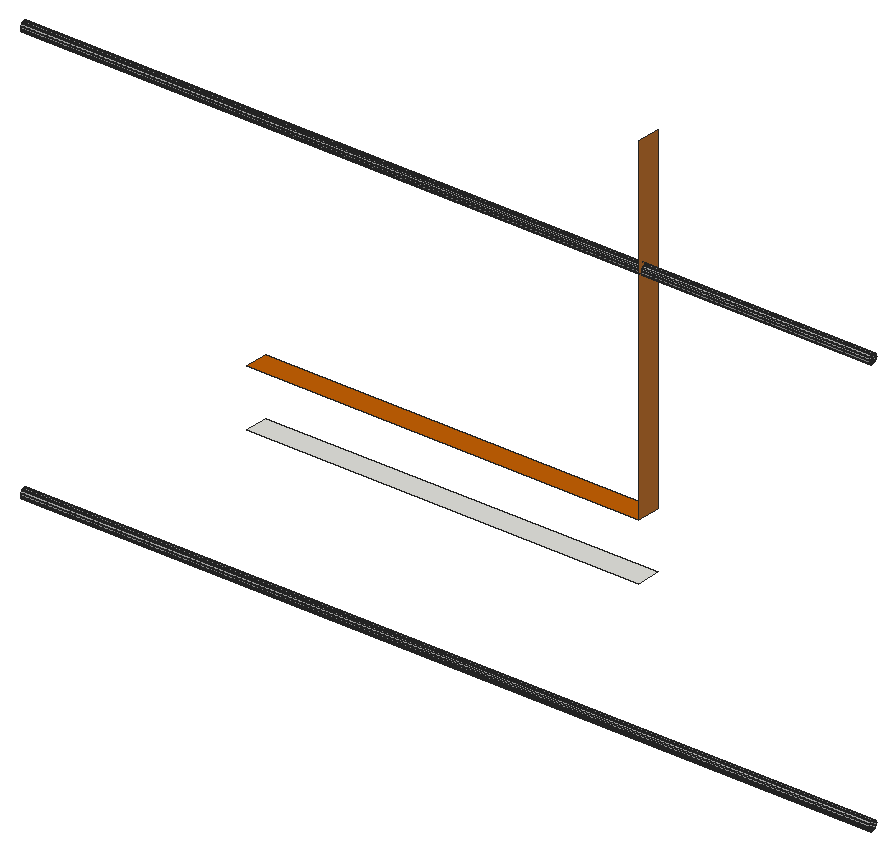
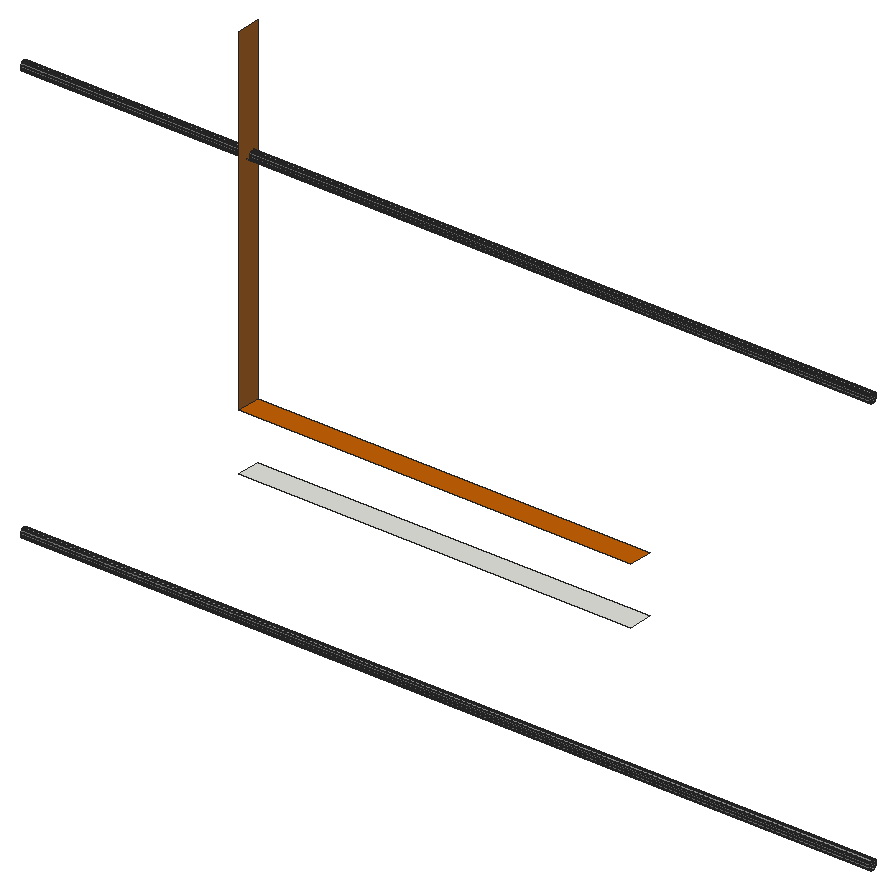
# SketchUp Ruby script. Lengths in inches.
U = 1.inch
M = Sketchup.active_model
def pt(a) = Geom::Point3d.new(a.map { |v| v * U })
def face(e, loops, mat)
  f = e.add_face(loops[0].map { |a| pt(a) })
  loops[1..].each { |l| e.add_face(l.map { |a| pt(a) }).erase! }
  f.material = f.back_material = mat if mat
  f
end
# faces: each face lists its corners as indices into pts; further lists are holes
def faces(e, pts, list, mat = nil) = list.each { |f| face(e, (f[0].is_a?(Array) ? f : [f]).map { |l| l.map { |i| pts[i] } }, mat) }
# xy, xz, yz: faces in a plane at the given z, y or x. An outline is a flat list of corners, or four numbers for a rectangle; further outlines are holes
def ring(l) = l.size == 4 ? [[l[0], l[1]], [l[2], l[1]], [l[2], l[3]], [l[0], l[3]]] : l.each_slice(2).to_a
def flat(e, list, mat, &to3) = list.each { |f| face(e, (f[0].is_a?(Array) ? f : [f]).map { |l| ring(l).map { |u, v| to3.(u, v) } }, mat) }
def xy(e, z, list, mat = nil) = flat(e, list, mat) { |x, y| [x, y, z] }
def xz(e, y, list, mat = nil) = flat(e, list, mat) { |x, z| [x, y, z] }
def yz(e, x, list, mat = nil) = flat(e, list, mat) { |y, z| [x, y, z] }
def lines(e, pts, list) = list.each { |a, b| e.add_line(pt(pts[a]), pt(pts[b])) }
# prism: a flat outline (further loops are holes) pulled along v
def prism(e, loops, v, mat = nil)
  f = face(e, loops, mat); d = Geom::Vector3d.new(v.map { |x| x * U })
  f.pushpull(f.normal.samedirection?(d) ? d.length : -d.length)
end
def box(e, o, s, mat = nil) = prism(e, [[o, [o[0] + s[0], o[1], o[2]], [o[0] + s[0], o[1] + s[1], o[2]], [o[0], o[1] + s[1], o[2]]]], [0, 0, s[2]], mat)
def at(x, y, z, deg = 0) = Geom::Transformation.translation(pt([x, y, z])) * Geom::Transformation.rotation(ORIGIN, Z_AXIS, deg.degrees)
def axes(o, x, y, z) = Geom::Transformation.new([*x, 0, *y, 0, *z, 0, *pt(o).to_a, 1])
def part(name) = M.definitions.add(name)
# library, detail: a bought-in or finely detailed component or shape, given as its bounding box
def library(name, o, s) = part(name).tap { |d| box(d.entities, o, s) }
def detail(e, o, s) = box(e.add_group.entities, o, s)
def put(e, d, t, mat = nil) = e.add_instance(d, t).tap { |i| i.material = mat if mat }
def group(e, t, mat = nil) = e.add_group.tap { |g| g.transformation = t; g.material = mat if mat }.entities
root = M.entities
M.materials.add("[0132_LightGray]").color = [169, 169, 169]
M.materials.add("[Wood Bamboo]").color = [195, 96, 5]
M.materials.add("[Wood Bamboo]1").color = [177, 105, 43]
xy(root,94.9,[[340.01,40.5625,381.26,43]])
xy(root,100.9,[[340.01,40.5625,381.26,43]],"[Wood Bamboo]")
yz(root,381.26,[[40.5625,100.9,43,136.59]],"[Wood Bamboo]1")
p = [[316.01,41.03,79.78],[316.01,41.15,79.73],[405.26,41.15,79.73],[405.26,41.03,79.78],[316.01,41.28,79.71],[405.26,41.28,79.71],
  [316.01,41.41,79.73],[405.26,41.41,79.73],[316.01,41.53,79.78],[405.26,41.53,79.78],[316.01,40.93,79.86],[405.26,40.93,79.86],
  [316.01,41.63,79.86],[405.26,41.63,79.86],[316.01,40.85,79.96],[405.26,40.85,79.96],[316.01,41.71,79.96],[405.26,41.71,79.96],
  [316.01,40.8,80.08],[405.26,40.8,80.08],[316.01,41.76,80.08],[405.26,41.76,80.08],[316.01,40.78,80.21],[405.26,40.78,80.21],
  [316.01,41.78,80.21],[405.26,41.78,80.21],[316.01,40.8,80.34],[405.26,40.8,80.34],[316.01,41.76,80.34],[405.26,41.76,80.34],
  [316.01,40.85,80.46],[405.26,40.85,80.46],[316.01,41.71,80.46],[405.26,41.71,80.46],[316.01,40.93,80.57],[405.26,40.93,80.57],
  [316.01,41.63,80.57],[405.26,41.63,80.57],[316.01,41.03,80.65],[405.26,41.03,80.65],[316.01,41.15,80.7],[405.26,41.15,80.7],
  [316.01,41.53,80.65],[316.01,41.41,80.7],[405.26,41.41,80.7],[405.26,41.53,80.65],[316.01,41.28,80.71],[405.26,41.28,80.71],
  [316.01,41.03,123.78],[316.01,41.15,123.73],[405.26,41.15,123.73],[405.26,41.03,123.78],[316.01,41.28,123.71],[405.26,41.28,123.71],
  [316.01,41.41,123.73],[405.26,41.41,123.73],[316.01,41.53,123.78],[405.26,41.53,123.78],[316.01,40.93,123.86],[405.26,40.93,123.86],
  [316.01,41.63,123.86],[405.26,41.63,123.86],[316.01,40.85,123.96],[405.26,40.85,123.96],[316.01,41.71,123.96],[405.26,41.71,123.96],
  [316.01,40.8,124.08],[405.26,40.8,124.08],[316.01,41.76,124.08],[405.26,41.76,124.08],[316.01,40.78,124.21],[405.26,40.78,124.21],
  [316.01,41.78,124.21],[405.26,41.78,124.21],[316.01,40.8,124.34],[405.26,40.8,124.34],[316.01,41.76,124.34],[405.26,41.76,124.34],
  [316.01,40.85,124.46],[405.26,40.85,124.46],[316.01,41.71,124.46],[405.26,41.71,124.46],[316.01,40.93,124.57],[405.26,40.93,124.57],
  [316.01,41.63,124.57],[405.26,41.63,124.57],[316.01,41.03,124.65],[405.26,41.03,124.65],[316.01,41.15,124.7],[405.26,41.15,124.7],
  [316.01,41.53,124.65],[316.01,41.41,124.7],[405.26,41.41,124.7],[405.26,41.53,124.65],[316.01,41.28,124.71],[405.26,41.28,124.71]]
faces(root,p,[[0,1,2,3],[1,4,5,2],[4,6,7,5],[6,8,9,7],[10,0,3,11],[8,12,13,9],[14,10,11,15],[12,16,17,13],
  [18,14,15,19],[16,20,21,17],[22,18,19,23],[20,24,25,21],[26,22,23,27],[24,28,29,25],[30,26,27,31],[28,32,33,29],
  [34,30,31,35],[32,36,37,33],[38,34,35,39],[40,38,39,41],[42,43,44,45],[36,42,45,37],[46,40,41,47],[43,46,47,44],
  [48,49,50,51],[49,52,53,50],[52,54,55,53],[54,56,57,55],[58,48,51,59],[56,60,61,57],[62,58,59,63],[60,64,65,61],
  [66,62,63,67],[64,68,69,65],[70,66,67,71],[68,72,73,69],[74,70,71,75],[72,76,77,73],[78,74,75,79],[76,80,81,77],
  [82,78,79,83],[80,84,85,81],[86,82,83,87],[88,86,87,89],[90,91,92,93],[84,90,93,85],[94,88,89,95],[91,94,95,92]],"[0132_LightGray]")
